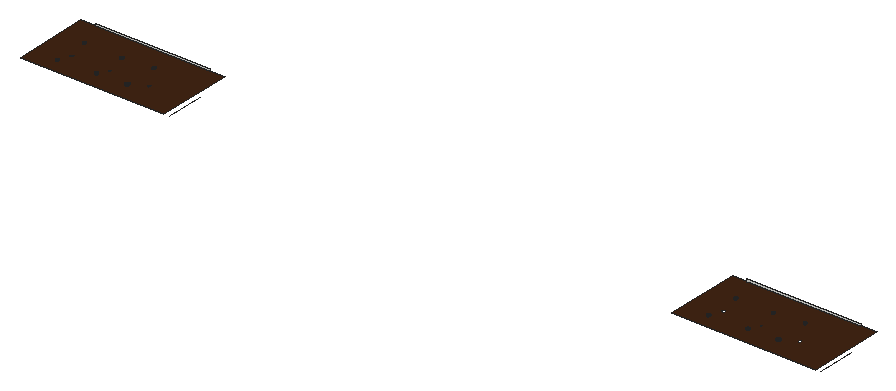
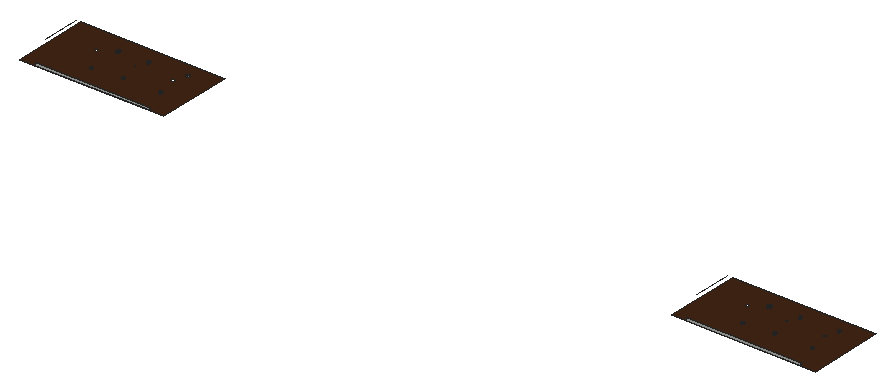
# SketchUp Ruby script. Lengths in inches.
U = 1.inch
M = Sketchup.active_model
def pt(a) = Geom::Point3d.new(a.map { |v| v * U })
def face(e, loops, mat)
  f = e.add_face(loops[0].map { |a| pt(a) })
  loops[1..].each { |l| e.add_face(l.map { |a| pt(a) }).erase! }
  f.material = f.back_material = mat if mat
  f
end
# faces: each face lists its corners as indices into pts; further lists are holes
def faces(e, pts, list, mat = nil) = list.each { |f| face(e, (f[0].is_a?(Array) ? f : [f]).map { |l| l.map { |i| pts[i] } }, mat) }
# xy, xz, yz: faces in a plane at the given z, y or x. An outline is a flat list of corners, or four numbers for a rectangle; further outlines are holes
def ring(l) = l.size == 4 ? [[l[0], l[1]], [l[2], l[1]], [l[2], l[3]], [l[0], l[3]]] : l.each_slice(2).to_a
def flat(e, list, mat, &to3) = list.each { |f| face(e, (f[0].is_a?(Array) ? f : [f]).map { |l| ring(l).map { |u, v| to3.(u, v) } }, mat) }
def xy(e, z, list, mat = nil) = flat(e, list, mat) { |x, y| [x, y, z] }
def xz(e, y, list, mat = nil) = flat(e, list, mat) { |x, z| [x, y, z] }
def yz(e, x, list, mat = nil) = flat(e, list, mat) { |y, z| [x, y, z] }
def lines(e, pts, list) = list.each { |a, b| e.add_line(pt(pts[a]), pt(pts[b])) }
# prism: a flat outline (further loops are holes) pulled along v
def prism(e, loops, v, mat = nil)
  f = face(e, loops, mat); d = Geom::Vector3d.new(v.map { |x| x * U })
  f.pushpull(f.normal.samedirection?(d) ? d.length : -d.length)
end
def box(e, o, s, mat = nil) = prism(e, [[o, [o[0] + s[0], o[1], o[2]], [o[0] + s[0], o[1] + s[1], o[2]], [o[0], o[1] + s[1], o[2]]]], [0, 0, s[2]], mat)
def at(x, y, z, deg = 0) = Geom::Transformation.translation(pt([x, y, z])) * Geom::Transformation.rotation(ORIGIN, Z_AXIS, deg.degrees)
def axes(o, x, y, z) = Geom::Transformation.new([*x, 0, *y, 0, *z, 0, *pt(o).to_a, 1])
def part(name) = M.definitions.add(name)
# library, detail: a bought-in or finely detailed component or shape, given as its bounding box
def library(name, o, s) = part(name).tap { |d| box(d.entities, o, s) }
def detail(e, o, s) = box(e.add_group.entities, o, s)
def put(e, d, t, mat = nil) = e.add_instance(d, t).tap { |i| i.material = mat if mat }
def group(e, t, mat = nil) = e.add_group.tap { |g| g.transformation = t; g.material = mat if mat }.entities
root = M.entities
M.materials.add("[Field Square Tile]").color = [211, 167, 108]
M.materials.add("[Wood Veneer 01]").color = [66, 38, 20]
xy(root,251.5,[[[232.96,2294.125,427.1,2396.68],[273.1,2327.89,273.89,2328,274.63,2328.3,275.26,2328.79,275.75,2329.43,276.06,2330.16,276.16,2330.96,276.06,2331.75,275.75,2332.49,275.26,2333.12,274.63,2333.61,273.89,2333.91,273.1,2334.02,272.31,2333.91,271.57,2333.61,270.93,2333.12,270.45,2332.49,270.14,2331.75,270.04,2330.96,270.14,2330.16,270.45,2329.43,270.93,2328.79,271.57,2328.3,272.31,2328],[377.04,2328.21,377.75,2328.3,378.42,2328.57,378.99,2329.01,379.42,2329.58,379.7,2330.24,379.79,2330.96,379.7,2331.67,379.42,2332.33,378.99,2332.9,378.42,2333.34,377.75,2333.61,377.04,2333.71,376.33,2333.61,375.67,2333.34,375.1,2332.9,374.66,2332.33,374.39,2331.67,374.29,2330.96,374.39,2330.24,374.66,2329.58,375.1,2329.01,375.67,2328.57,376.33,2328.3],[324.47,2328.39,325.13,2328.48,325.75,2328.74,326.28,2329.14,326.69,2329.68,326.95,2330.29,327.03,2330.96,326.95,2331.62,326.69,2332.24,326.28,2332.77,325.75,2333.18,325.13,2333.43,324.47,2333.52,323.81,2333.43,323.19,2333.18,322.66,2332.77,322.25,2332.24,322,2331.62,321.91,2330.96,322,2330.29,322.25,2329.68,322.66,2329.14,323.19,2328.74,323.81,2328.48],[357.2,2316.65,357.83,2316.73,358.42,2316.97,358.92,2317.36,359.31,2317.87,359.55,2318.45,359.63,2319.08,359.55,2319.72,359.31,2320.3,358.92,2320.81,358.42,2321.2,357.83,2321.4375,357.2,2321.52,356.57,2321.4375,355.98,2321.2,355.47,2320.81,355.09,2320.3,354.84,2319.72,354.76,2319.08,354.84,2318.45,355.09,2317.87,355.47,2317.36,355.98,2316.97,356.57,2316.73],[266.8,2358.2,267.28,2358.27,267.74,2358.46,268.125,2358.75,268.42,2359.14,268.61,2359.59,268.67,2360.08,268.61,2360.56,268.42,2361.02,268.125,2361.41,267.74,2361.7,267.28,2361.89,266.8,2361.95,266.3125,2361.89,265.86,2361.7,265.47,2361.41,265.17,2361.02,264.99,2360.56,264.92,2360.08,264.99,2359.59,265.17,2359.14,265.47,2358.75,265.86,2358.46,266.3125,2358.27],[317.24,2358.2,317.72,2358.27,318.17,2358.46,318.5625,2358.75,318.86,2359.14,319.05,2359.59,319.11,2360.08,319.05,2360.56,318.86,2361.02,318.5625,2361.41,318.17,2361.7,317.72,2361.89,317.24,2361.95,316.75,2361.89,316.3,2361.7,315.91,2361.41,315.61,2361.02,315.42,2360.56,315.36,2360.08,315.42,2359.59,315.61,2359.14,315.91,2358.75,316.3,2358.46,316.75,2358.27],[317.24,2315.39,317.72,2315.46,318.17,2315.64,318.5625,2315.94,318.86,2316.33,319.05,2316.78,319.11,2317.27,319.05,2317.75,318.86,2318.2,318.5625,2318.59,318.17,2318.89,317.72,2319.08,317.24,2319.14,316.75,2319.08,316.3,2318.89,315.91,2318.59,315.61,2318.2,315.42,2317.75,315.36,2317.27,315.42,2316.78,315.61,2316.33,315.91,2315.94,316.3,2315.64,316.75,2315.46],[266.8,2312.27,267.28,2312.33,267.74,2312.52,268.125,2312.82,268.42,2313.2,268.61,2313.66,268.67,2314.14,268.61,2314.63,268.42,2315.08,268.125,2315.47,267.74,2315.77,267.28,2315.95,266.8,2316.02,266.3125,2315.95,265.86,2315.77,265.47,2315.47,265.17,2315.08,264.99,2314.63,264.92,2314.14,264.99,2313.66,265.17,2313.2,265.47,2312.82,265.86,2312.52,266.3125,2312.33],[357.2,2362.38,357.63,2362.4375,358.04,2362.6,358.39,2362.87,358.66,2363.22,358.83,2363.63,358.88,2364.07,358.83,2364.5,358.66,2364.91,358.39,2365.26,358.04,2365.53,357.63,2365.7,357.2,2365.75,356.76,2365.7,356.35,2365.53,356,2365.26,355.74,2364.91,355.57,2364.5,355.51,2364.07,355.57,2363.63,355.74,2363.22,356,2362.87,356.35,2362.6,356.76,2362.4375]],[[1111.71,2294.125,1305.85,2396.68],[1151.85,2327.89,1152.64,2328,1153.38,2328.3,1154.01,2328.79,1154.5,2329.43,1154.81,2330.16,1154.91,2330.96,1154.81,2331.75,1154.5,2332.49,1154.01,2333.12,1153.38,2333.61,1152.64,2333.91,1151.85,2334.02,1151.06,2333.91,1150.32,2333.61,1149.68,2333.12,1149.2,2332.49,1148.89,2331.75,1148.79,2330.96,1148.89,2330.16,1149.2,2329.43,1149.68,2328.79,1150.32,2328.3,1151.06,2328],[1255.79,2328.21,1256.5,2328.3,1257.17,2328.57,1257.74,2329.01,1258.17,2329.58,1258.45,2330.24,1258.54,2330.96,1258.45,2331.67,1258.17,2332.33,1257.74,2332.9,1257.17,2333.34,1256.5,2333.61,1255.79,2333.71,1255.08,2333.61,1254.42,2333.34,1253.85,2332.9,1253.41,2332.33,1253.14,2331.67,1253.04,2330.96,1253.14,2330.24,1253.41,2329.58,1253.85,2329.01,1254.42,2328.57,1255.08,2328.3],[1203.22,2328.39,1203.88,2328.48,1204.5,2328.74,1205.03,2329.14,1205.44,2329.68,1205.7,2330.29,1205.78,2330.96,1205.7,2331.62,1205.44,2332.24,1205.03,2332.77,1204.5,2333.18,1203.88,2333.43,1203.22,2333.52,1202.56,2333.43,1201.94,2333.18,1201.41,2332.77,1201,2332.24,1200.75,2331.62,1200.66,2330.96,1200.75,2330.29,1201,2329.68,1201.41,2329.14,1201.94,2328.74,1202.56,2328.48],[1235.95,2316.65,1236.58,2316.73,1237.17,2316.97,1237.67,2317.36,1238.06,2317.87,1238.3,2318.45,1238.38,2319.08,1238.3,2319.72,1238.06,2320.3,1237.67,2320.81,1237.17,2321.2,1236.58,2321.4375,1235.95,2321.52,1235.32,2321.4375,1234.73,2321.2,1234.22,2320.81,1233.84,2320.3,1233.59,2319.72,1233.51,2319.08,1233.59,2318.45,1233.84,2317.87,1234.22,2317.36,1234.73,2316.97,1235.32,2316.73],[1145.55,2358.2,1146.03,2358.27,1146.49,2358.46,1146.875,2358.75,1147.17,2359.14,1147.36,2359.59,1147.42,2360.08,1147.36,2360.56,1147.17,2361.02,1146.875,2361.41,1146.49,2361.7,1146.03,2361.89,1145.55,2361.95,1145.0625,2361.89,1144.61,2361.7,1144.22,2361.41,1143.92,2361.02,1143.74,2360.56,1143.67,2360.08,1143.74,2359.59,1143.92,2359.14,1144.22,2358.75,1144.61,2358.46,1145.0625,2358.27],[1195.99,2358.2,1196.47,2358.27,1196.92,2358.46,1197.3125,2358.75,1197.61,2359.14,1197.8,2359.59,1197.86,2360.08,1197.8,2360.56,1197.61,2361.02,1197.3125,2361.41,1196.92,2361.7,1196.47,2361.89,1195.99,2361.95,1195.5,2361.89,1195.05,2361.7,1194.66,2361.41,1194.36,2361.02,1194.17,2360.56,1194.11,2360.08,1194.17,2359.59,1194.36,2359.14,1194.66,2358.75,1195.05,2358.46,1195.5,2358.27],[1195.99,2315.39,1196.47,2315.46,1196.92,2315.64,1197.3125,2315.94,1197.61,2316.33,1197.8,2316.78,1197.86,2317.27,1197.8,2317.75,1197.61,2318.2,1197.3125,2318.59,1196.92,2318.89,1196.47,2319.08,1195.99,2319.14,1195.5,2319.08,1195.05,2318.89,1194.66,2318.59,1194.36,2318.2,1194.17,2317.75,1194.11,2317.27,1194.17,2316.78,1194.36,2316.33,1194.66,2315.94,1195.05,2315.64,1195.5,2315.46],[1145.55,2312.27,1146.03,2312.33,1146.49,2312.52,1146.875,2312.82,1147.17,2313.2,1147.36,2313.66,1147.42,2314.14,1147.36,2314.63,1147.17,2315.08,1146.875,2315.47,1146.49,2315.77,1146.03,2315.95,1145.55,2316.02,1145.0625,2315.95,1144.61,2315.77,1144.22,2315.47,1143.92,2315.08,1143.74,2314.63,1143.67,2314.14,1143.74,2313.66,1143.92,2313.2,1144.22,2312.82,1144.61,2312.52,1145.0625,2312.33],[1235.95,2362.38,1236.38,2362.4375,1236.79,2362.6,1237.14,2362.87,1237.41,2363.22,1237.58,2363.63,1237.63,2364.07,1237.58,2364.5,1237.41,2364.91,1237.14,2365.26,1236.79,2365.53,1236.38,2365.7,1235.95,2365.75,1235.51,2365.7,1235.1,2365.53,1234.75,2365.26,1234.49,2364.91,1234.32,2364.5,1234.26,2364.07,1234.32,2363.63,1234.49,2363.22,1234.75,2362.87,1235.1,2362.6,1235.51,2362.4375]]],"[Wood Veneer 01]")
xz(root,2396.68,[[252.78,251.5,252.84,254.5],[252.84,251.5,406.85,254.5],[1131.53,251.5,1131.59,254.5],[1131.59,251.5,1285.6,254.5]])
p = [[266.3125,2312.33,251.5],[265.86,2312.52,251.5],[265.86,2312.52,252.5],[266.3125,2312.33,252.5],[266.8,2312.27,251.5],[266.8,2312.27,252.5],
  [267.28,2312.33,251.5],[267.28,2312.33,252.5],[267.74,2312.52,251.5],[267.74,2312.52,252.5],[1145.0625,2312.33,251.5],[1144.61,2312.52,251.5],
  [1144.61,2312.52,252.5],[1145.0625,2312.33,252.5],[1145.55,2312.27,251.5],[1145.55,2312.27,252.5],[1146.03,2312.33,251.5],[1146.03,2312.33,252.5],
  [1146.49,2312.52,251.5],[1146.49,2312.52,252.5],[265.47,2312.82,251.5],[265.47,2312.82,252.5],[268.125,2312.82,251.5],[268.125,2312.82,252.5],
  [1144.22,2312.82,251.5],[1144.22,2312.82,252.5],[1146.875,2312.82,251.5],[1146.875,2312.82,252.5],[265.17,2313.2,251.5],[265.17,2313.2,252.5],
  [268.42,2313.2,251.5],[268.42,2313.2,252.5],[1143.92,2313.2,251.5],[1143.92,2313.2,252.5],[1147.17,2313.2,251.5],[1147.17,2313.2,252.5],
  [264.99,2313.66,251.5],[264.99,2313.66,252.5],[268.61,2313.66,251.5],[268.61,2313.66,252.5],[1143.74,2313.66,251.5],[1143.74,2313.66,252.5],
  [1147.36,2313.66,251.5],[1147.36,2313.66,252.5],[264.92,2314.14,251.5],[264.92,2314.14,252.5],[268.67,2314.14,251.5],[268.67,2314.14,252.5],
  [1143.67,2314.14,251.5],[1143.67,2314.14,252.5],[1147.42,2314.14,251.5],[1147.42,2314.14,252.5],[264.99,2314.63,251.5],[264.99,2314.63,252.5],
  [268.61,2314.63,251.5],[268.61,2314.63,252.5],[1143.74,2314.63,251.5],[1143.74,2314.63,252.5],[1147.36,2314.63,251.5],[1147.36,2314.63,252.5],
  [265.17,2315.08,251.5],[265.17,2315.08,252.5],[268.42,2315.08,251.5],[268.42,2315.08,252.5],[1143.92,2315.08,251.5],[1143.92,2315.08,252.5],
  [1147.17,2315.08,251.5],[1147.17,2315.08,252.5],[265.47,2315.47,251.5],[265.47,2315.47,252.5],[268.125,2315.47,251.5],[268.125,2315.47,252.5],
  [1144.22,2315.47,251.5],[1144.22,2315.47,252.5],[1146.875,2315.47,251.5],[1146.875,2315.47,252.5],[317.24,2315.39,251.5],[316.75,2315.46,251.5],
  [316.75,2315.46,252.5],[317.24,2315.39,252.5],[317.72,2315.46,251.5],[317.72,2315.46,252.5],[1195.99,2315.39,251.5],[1195.5,2315.46,251.5],
  [1195.5,2315.46,252.5],[1195.99,2315.39,252.5],[1196.47,2315.46,251.5],[1196.47,2315.46,252.5],[265.86,2315.77,251.5],[265.86,2315.77,252.5],
  [267.74,2315.77,251.5],[267.74,2315.77,252.5],[316.3,2315.64,251.5],[316.3,2315.64,252.5],[318.17,2315.64,251.5],[318.17,2315.64,252.5],
  [1144.61,2315.77,251.5],[1144.61,2315.77,252.5],[1146.49,2315.77,251.5],[1146.49,2315.77,252.5],[1195.05,2315.64,251.5],[1195.05,2315.64,252.5],
  [1196.92,2315.64,251.5],[1196.92,2315.64,252.5],[315.91,2315.94,251.5],[315.91,2315.94,252.5],[318.5625,2315.94,251.5],[318.5625,2315.94,252.5],
  [1194.66,2315.94,251.5],[1194.66,2315.94,252.5],[1197.3125,2315.94,251.5],[1197.3125,2315.94,252.5],[266.3125,2315.95,251.5],[266.3125,2315.95,252.5],
  [267.28,2315.95,251.5],[267.28,2315.95,252.5],[1145.0625,2315.95,251.5],[1145.0625,2315.95,252.5],[1146.03,2315.95,251.5],[1146.03,2315.95,252.5],
  [315.61,2316.33,251.5],[315.61,2316.33,252.5],[318.86,2316.33,251.5],[318.86,2316.33,252.5],[1194.36,2316.33,251.5],[1194.36,2316.33,252.5],
  [1197.61,2316.33,251.5],[1197.61,2316.33,252.5],[266.8,2316.02,251.5],[266.8,2316.02,252.5],[1145.55,2316.02,251.5],[1145.55,2316.02,252.5],
  [315.42,2316.78,251.5],[315.42,2316.78,252.5],[319.05,2316.78,251.5],[319.05,2316.78,252.5],[1194.17,2316.78,251.5],[1194.17,2316.78,252.5],
  [1197.8,2316.78,251.5],[1197.8,2316.78,252.5],[357.2,2316.65,251.5],[356.57,2316.73,251.5],[356.57,2316.73,252.5625],[357.2,2316.65,252.5625],
  [357.83,2316.73,251.5],[357.83,2316.73,252.5625],[1235.95,2316.65,251.5],[1235.32,2316.73,251.5],[1235.32,2316.73,252.5625],[1235.95,2316.65,252.5625],
  [1236.58,2316.73,251.5],[1236.58,2316.73,252.5625],[355.98,2316.97,251.5],[355.98,2316.97,252.5625],[358.42,2316.97,251.5],[358.42,2316.97,252.5625],
  [1234.73,2316.97,251.5],[1234.73,2316.97,252.5625],[1237.17,2316.97,251.5],[1237.17,2316.97,252.5625],[315.36,2317.27,251.5],[315.36,2317.27,252.5],
  [319.11,2317.27,251.5],[319.11,2317.27,252.5],[1194.11,2317.27,251.5],[1194.11,2317.27,252.5],[1197.86,2317.27,251.5],[1197.86,2317.27,252.5],
  [355.47,2317.36,251.5],[355.47,2317.36,252.5625],[358.92,2317.36,251.5],[358.92,2317.36,252.5625],[1234.22,2317.36,251.5],[1234.22,2317.36,252.5625],
  [1237.67,2317.36,251.5],[1237.67,2317.36,252.5625],[315.42,2317.75,251.5],[315.42,2317.75,252.5],[319.05,2317.75,251.5],[319.05,2317.75,252.5],
  [1194.17,2317.75,251.5],[1194.17,2317.75,252.5],[1197.8,2317.75,251.5],[1197.8,2317.75,252.5],[355.09,2317.87,251.5],[355.09,2317.87,252.5625],
  [359.31,2317.87,251.5],[359.31,2317.87,252.5625],[1233.84,2317.87,251.5],[1233.84,2317.87,252.5625],[1238.06,2317.87,251.5],[1238.06,2317.87,252.5625],
  [315.61,2318.2,251.5],[315.61,2318.2,252.5],[318.86,2318.2,251.5],[318.86,2318.2,252.5],[1194.36,2318.2,251.5],[1194.36,2318.2,252.5],
  [1197.61,2318.2,251.5],[1197.61,2318.2,252.5],[354.84,2318.45,251.5],[354.84,2318.45,252.5625],[359.55,2318.45,251.5],[359.55,2318.45,252.5625],
  [1233.59,2318.45,251.5],[1233.59,2318.45,252.5625],[1238.3,2318.45,251.5],[1238.3,2318.45,252.5625],[315.91,2318.59,251.5],[315.91,2318.59,252.5],
  [318.5625,2318.59,251.5],[318.5625,2318.59,252.5],[1194.66,2318.59,251.5],[1194.66,2318.59,252.5],[1197.3125,2318.59,251.5],[1197.3125,2318.59,252.5],
  [354.76,2319.08,251.5],[354.76,2319.08,252.5625],[359.63,2319.08,251.5],[359.63,2319.08,252.5625],[1233.51,2319.08,251.5],[1233.51,2319.08,252.5625],
  [1238.38,2319.08,251.5],[1238.38,2319.08,252.5625],[316.3,2318.89,251.5],[316.3,2318.89,252.5],[318.17,2318.89,251.5],[318.17,2318.89,252.5],
  [1195.05,2318.89,251.5],[1195.05,2318.89,252.5],[1196.92,2318.89,251.5],[1196.92,2318.89,252.5],[316.75,2319.08,251.5],[316.75,2319.08,252.5],
  [317.72,2319.08,251.5],[317.72,2319.08,252.5],[1195.5,2319.08,251.5],[1195.5,2319.08,252.5],[1196.47,2319.08,251.5],[1196.47,2319.08,252.5],
  [317.24,2319.14,251.5],[317.24,2319.14,252.5],[354.84,2319.72,251.5],[354.84,2319.72,252.5625],[359.55,2319.72,251.5],[359.55,2319.72,252.5625],
  [1195.99,2319.14,251.5],[1195.99,2319.14,252.5],[1233.59,2319.72,251.5],[1233.59,2319.72,252.5625],[1238.3,2319.72,251.5],[1238.3,2319.72,252.5625],
  [355.09,2320.3,251.5],[355.09,2320.3,252.5625],[359.31,2320.3,251.5],[359.31,2320.3,252.5625],[1233.84,2320.3,251.5],[1233.84,2320.3,252.5625],
  [1238.06,2320.3,251.5],[1238.06,2320.3,252.5625],[355.47,2320.81,251.5],[355.47,2320.81,252.5625],[358.92,2320.81,251.5],[358.92,2320.81,252.5625],
  [1234.22,2320.81,251.5],[1234.22,2320.81,252.5625],[1237.67,2320.81,251.5],[1237.67,2320.81,252.5625],[355.98,2321.2,251.5],[355.98,2321.2,252.5625],
  [358.42,2321.2,251.5],[358.42,2321.2,252.5625],[1234.73,2321.2,251.5],[1234.73,2321.2,252.5625],[1237.17,2321.2,251.5],[1237.17,2321.2,252.5625],
  [356.57,2321.4375,251.5],[356.57,2321.4375,252.5625],[357.83,2321.4375,251.5],[357.83,2321.4375,252.5625],[1235.32,2321.4375,251.5],[1235.32,2321.4375,252.5625],
  [1236.58,2321.4375,251.5],[1236.58,2321.4375,252.5625],[357.2,2321.52,251.5],[357.2,2321.52,252.5625],[1235.95,2321.52,251.5],[1235.95,2321.52,252.5625],
  [266.8,2358.2,251.5],[266.3125,2358.27,251.5],[266.3125,2358.27,252.5],[266.8,2358.2,252.5],[267.28,2358.27,251.5],[267.28,2358.27,252.5],
  [317.24,2358.2,251.5],[316.75,2358.27,251.5],[316.75,2358.27,252.5],[317.24,2358.2,252.5],[317.72,2358.27,251.5],[317.72,2358.27,252.5],
  [1145.55,2358.2,251.5],[1145.0625,2358.27,251.5],[1145.0625,2358.27,252.5],[1145.55,2358.2,252.5],[1146.03,2358.27,251.5],[1146.03,2358.27,252.5],
  [1195.99,2358.2,251.5],[1195.5,2358.27,251.5],[1195.5,2358.27,252.5],[1195.99,2358.2,252.5],[1196.47,2358.27,251.5],[1196.47,2358.27,252.5],
  [265.86,2358.46,251.5],[265.86,2358.46,252.5],[267.74,2358.46,251.5],[267.74,2358.46,252.5],[316.3,2358.46,251.5],[316.3,2358.46,252.5],
  [318.17,2358.46,251.5],[318.17,2358.46,252.5],[1144.61,2358.46,251.5],[1144.61,2358.46,252.5],[1146.49,2358.46,251.5],[1146.49,2358.46,252.5],
  [1195.05,2358.46,251.5],[1195.05,2358.46,252.5],[1196.92,2358.46,251.5],[1196.92,2358.46,252.5],[265.47,2358.75,251.5],[265.47,2358.75,252.5],
  [268.125,2358.75,251.5],[268.125,2358.75,252.5],[315.91,2358.75,251.5],[315.91,2358.75,252.5],[318.5625,2358.75,251.5],[318.5625,2358.75,252.5],
  [1144.22,2358.75,251.5],[1144.22,2358.75,252.5],[1146.875,2358.75,251.5],[1146.875,2358.75,252.5],[1194.66,2358.75,251.5],[1194.66,2358.75,252.5],
  [1197.3125,2358.75,251.5],[1197.3125,2358.75,252.5],[265.17,2359.14,251.5],[265.17,2359.14,252.5],[268.42,2359.14,251.5],[268.42,2359.14,252.5],
  [315.61,2359.14,251.5],[315.61,2359.14,252.5],[318.86,2359.14,251.5],[318.86,2359.14,252.5],[1143.92,2359.14,251.5],[1143.92,2359.14,252.5],
  [1147.17,2359.14,251.5],[1147.17,2359.14,252.5],[1194.36,2359.14,251.5],[1194.36,2359.14,252.5],[1197.61,2359.14,251.5],[1197.61,2359.14,252.5],
  [264.99,2359.59,251.5],[264.99,2359.59,252.5],[268.61,2359.59,251.5],[268.61,2359.59,252.5],[315.42,2359.59,251.5],[315.42,2359.59,252.5],
  [319.05,2359.59,251.5],[319.05,2359.59,252.5],[1143.74,2359.59,251.5],[1143.74,2359.59,252.5],[1147.36,2359.59,251.5],[1147.36,2359.59,252.5],
  [1194.17,2359.59,251.5],[1194.17,2359.59,252.5],[1197.8,2359.59,251.5],[1197.8,2359.59,252.5],[264.92,2360.08,251.5],[264.92,2360.08,252.5],
  [268.67,2360.08,251.5],[268.67,2360.08,252.5],[315.36,2360.08,251.5],[315.36,2360.08,252.5],[319.11,2360.08,251.5],[319.11,2360.08,252.5],
  [1143.67,2360.08,251.5],[1143.67,2360.08,252.5],[1147.42,2360.08,251.5],[1147.42,2360.08,252.5],[1194.11,2360.08,251.5],[1194.11,2360.08,252.5],
  [1197.86,2360.08,251.5],[1197.86,2360.08,252.5],[264.99,2360.56,251.5],[264.99,2360.56,252.5],[268.61,2360.56,251.5],[268.61,2360.56,252.5],
  [315.42,2360.56,251.5],[315.42,2360.56,252.5],[319.05,2360.56,251.5],[319.05,2360.56,252.5],[1143.74,2360.56,251.5],[1143.74,2360.56,252.5],
  [1147.36,2360.56,251.5],[1147.36,2360.56,252.5],[1194.17,2360.56,251.5],[1194.17,2360.56,252.5],[1197.8,2360.56,251.5],[1197.8,2360.56,252.5],
  [265.17,2361.02,251.5],[265.17,2361.02,252.5],[268.42,2361.02,251.5],[268.42,2361.02,252.5],[315.61,2361.02,251.5],[315.61,2361.02,252.5],
  [318.86,2361.02,251.5],[318.86,2361.02,252.5],[1143.92,2361.02,251.5],[1143.92,2361.02,252.5],[1147.17,2361.02,251.5],[1147.17,2361.02,252.5],
  [1194.36,2361.02,251.5],[1194.36,2361.02,252.5],[1197.61,2361.02,251.5],[1197.61,2361.02,252.5],[265.47,2361.41,251.5],[265.47,2361.41,252.5],
  [268.125,2361.41,251.5],[268.125,2361.41,252.5],[315.91,2361.41,251.5],[315.91,2361.41,252.5],[318.5625,2361.41,251.5],[318.5625,2361.41,252.5],
  [1144.22,2361.41,251.5],[1144.22,2361.41,252.5],[1146.875,2361.41,251.5],[1146.875,2361.41,252.5],[1194.66,2361.41,251.5],[1194.66,2361.41,252.5],
  [1197.3125,2361.41,251.5],[1197.3125,2361.41,252.5],[265.86,2361.7,251.5],[265.86,2361.7,252.5],[267.74,2361.7,251.5],[267.74,2361.7,252.5],
  [316.3,2361.7,251.5],[316.3,2361.7,252.5],[318.17,2361.7,251.5],[318.17,2361.7,252.5],[1144.61,2361.7,251.5],[1144.61,2361.7,252.5],
  [1146.49,2361.7,251.5],[1146.49,2361.7,252.5],[1195.05,2361.7,251.5],[1195.05,2361.7,252.5],[1196.92,2361.7,251.5],[1196.92,2361.7,252.5],
  [266.3125,2361.89,251.5],[266.3125,2361.89,252.5],[267.28,2361.89,251.5],[267.28,2361.89,252.5],[316.75,2361.89,251.5],[316.75,2361.89,252.5],
  [317.72,2361.89,251.5],[317.72,2361.89,252.5],[1145.0625,2361.89,251.5],[1145.0625,2361.89,252.5],[1146.03,2361.89,251.5],[1146.03,2361.89,252.5],
  [1195.5,2361.89,251.5],[1195.5,2361.89,252.5],[1196.47,2361.89,251.5],[1196.47,2361.89,252.5],[266.8,2361.95,251.5],[266.8,2361.95,252.5],
  [317.24,2361.95,251.5],[317.24,2361.95,252.5],[1145.55,2361.95,251.5],[1145.55,2361.95,252.5],[1195.99,2361.95,251.5],[1195.99,2361.95,252.5],
  [356.76,2362.4375,251.5],[356.35,2362.6,251.5],[356.35,2362.6,252.4375],[356.76,2362.4375,252.4375],[357.2,2362.38,251.5],[357.2,2362.38,252.4375],
  [357.63,2362.4375,251.5],[357.63,2362.4375,252.4375],[358.04,2362.6,251.5],[358.04,2362.6,252.4375],[1235.51,2362.4375,251.5],[1235.1,2362.6,251.5],
  [1235.1,2362.6,252.4375],[1235.51,2362.4375,252.4375],[1235.95,2362.38,251.5],[1235.95,2362.38,252.4375],[1236.38,2362.4375,251.5],[1236.38,2362.4375,252.4375],
  [1236.79,2362.6,251.5],[1236.79,2362.6,252.4375],[356,2362.87,251.5],[356,2362.87,252.4375],[358.39,2362.87,251.5],[358.39,2362.87,252.4375],
  [1234.75,2362.87,251.5],[1234.75,2362.87,252.4375],[1237.14,2362.87,251.5],[1237.14,2362.87,252.4375],[355.74,2363.22,251.5],[355.74,2363.22,252.4375],
  [358.66,2363.22,251.5],[358.66,2363.22,252.4375],[1234.49,2363.22,251.5],[1234.49,2363.22,252.4375],[1237.41,2363.22,251.5],[1237.41,2363.22,252.4375],
  [355.57,2363.63,251.5],[355.57,2363.63,252.4375],[358.83,2363.63,251.5],[358.83,2363.63,252.4375],[1234.32,2363.63,251.5],[1234.32,2363.63,252.4375],
  [1237.58,2363.63,251.5],[1237.58,2363.63,252.4375],[355.51,2364.07,251.5],[355.51,2364.07,252.4375],[358.88,2364.07,251.5],[358.88,2364.07,252.4375],
  [1234.26,2364.07,251.5],[1234.26,2364.07,252.4375],[1237.63,2364.07,251.5],[1237.63,2364.07,252.4375],[355.57,2364.5,251.5],[355.57,2364.5,252.4375],
  [358.83,2364.5,251.5],[358.83,2364.5,252.4375],[1234.32,2364.5,251.5],[1234.32,2364.5,252.4375],[1237.58,2364.5,251.5],[1237.58,2364.5,252.4375],
  [355.74,2364.91,251.5],[355.74,2364.91,252.4375],[358.66,2364.91,251.5],[358.66,2364.91,252.4375],[1234.49,2364.91,251.5],[1234.49,2364.91,252.4375],
  [1237.41,2364.91,251.5],[1237.41,2364.91,252.4375],[356,2365.26,251.5],[356,2365.26,252.4375],[358.39,2365.26,251.5],[358.39,2365.26,252.4375],
  [1234.75,2365.26,251.5],[1234.75,2365.26,252.4375],[1237.14,2365.26,251.5],[1237.14,2365.26,252.4375],[356.35,2365.53,251.5],[356.35,2365.53,252.4375],
  [358.04,2365.53,251.5],[358.04,2365.53,252.4375],[1235.1,2365.53,251.5],[1235.1,2365.53,252.4375],[1236.79,2365.53,251.5],[1236.79,2365.53,252.4375],
  [356.76,2365.7,251.5],[356.76,2365.7,252.4375],[357.63,2365.7,251.5],[357.63,2365.7,252.4375],[1235.51,2365.7,251.5],[1235.51,2365.7,252.4375],
  [1236.38,2365.7,251.5],[1236.38,2365.7,252.4375],[357.2,2365.75,251.5],[357.2,2365.75,252.4375],[1235.95,2365.75,251.5],[1235.95,2365.75,252.4375],
  [433.97,2346.71,251.5],[433.97,2294.125,251.5],[1312.72,2346.71,251.5],[1312.72,2294.125,251.5]]
faces(root,p,[[0,1,2,3],[4,0,3,5],[6,4,5,7],[8,6,7,9],[10,11,12,13],[14,10,13,15],[16,14,15,17],[18,16,17,19],
  [1,20,21,2],[22,8,9,23],[11,24,25,12],[26,18,19,27],[20,28,29,21],[30,22,23,31],[24,32,33,25],[34,26,27,35],
  [28,36,37,29],[38,30,31,39],[32,40,41,33],[42,34,35,43],[36,44,45,37],[46,38,39,47],[40,48,49,41],[50,42,43,51],
  [44,52,53,45],[54,46,47,55],[48,56,57,49],[58,50,51,59],[52,60,61,53],[62,54,55,63],[56,64,65,57],[66,58,59,67],
  [60,68,69,61],[70,62,63,71],[64,72,73,65],[74,66,67,75],[76,77,78,79],[80,76,79,81],[82,83,84,85],[86,82,85,87],
  [68,88,89,69],[90,70,71,91],[77,92,93,78],[94,80,81,95],[72,96,97,73],[98,74,75,99],[83,100,101,84],[102,86,87,103],
  [92,104,105,93],[106,94,95,107],[100,108,109,101],[110,102,103,111],[88,112,113,89],[114,90,91,115],[96,116,117,97],[118,98,99,119],
  [104,120,121,105],[122,106,107,123],[108,124,125,109],[126,110,111,127],[112,128,129,113],[128,114,115,129],[116,130,131,117],[130,118,119,131],
  [120,132,133,121],[134,122,123,135],[124,136,137,125],[138,126,127,139],[140,141,142,143],[144,140,143,145],[146,147,148,149],[150,146,149,151],
  [141,152,153,142],[154,144,145,155],[147,156,157,148],[158,150,151,159],[132,160,161,133],[162,134,135,163],[136,164,165,137],[166,138,139,167],
  [152,168,169,153],[170,154,155,171],[156,172,173,157],[174,158,159,175],[160,176,177,161],[178,162,163,179],[164,180,181,165],[182,166,167,183],
  [168,184,185,169],[186,170,171,187],[172,188,189,173],[190,174,175,191],[176,192,193,177],[194,178,179,195],[180,196,197,181],[198,182,183,199],
  [184,200,201,185],[202,186,187,203],[188,204,205,189],[206,190,191,207],[192,208,209,193],[210,194,195,211],[196,212,213,197],[214,198,199,215],
  [200,216,217,201],[218,202,203,219],[204,220,221,205],[222,206,207,223],[208,224,225,209],[226,210,211,227],[212,228,229,213],[230,214,215,231],
  [224,232,233,225],[234,226,227,235],[228,236,237,229],[238,230,231,239],[232,240,241,233],[240,234,235,241],[216,242,243,217],[244,218,219,245],
  [236,246,247,237],[246,238,239,247],[220,248,249,221],[250,222,223,251],[242,252,253,243],[254,244,245,255],[248,256,257,249],[258,250,251,259],
  [252,260,261,253],[262,254,255,263],[256,264,265,257],[266,258,259,267],[260,268,269,261],[270,262,263,271],[264,272,273,265],[274,266,267,275],
  [268,276,277,269],[278,270,271,279],[272,280,281,273],[282,274,275,283],[276,284,285,277],[284,278,279,285],[280,286,287,281],[286,282,283,287],
  [288,289,290,291],[292,288,291,293],[294,295,296,297],[298,294,297,299],[300,301,302,303],[304,300,303,305],[306,307,308,309],[310,306,309,311],
  [289,312,313,290],[314,292,293,315],[295,316,317,296],[318,298,299,319],[301,320,321,302],[322,304,305,323],[307,324,325,308],[326,310,311,327],
  [312,328,329,313],[330,314,315,331],[316,332,333,317],[334,318,319,335],[320,336,337,321],[338,322,323,339],[324,340,341,325],[342,326,327,343],
  [328,344,345,329],[346,330,331,347],[332,348,349,333],[350,334,335,351],[336,352,353,337],[354,338,339,355],[340,356,357,341],[358,342,343,359],
  [344,360,361,345],[362,346,347,363],[348,364,365,349],[366,350,351,367],[352,368,369,353],[370,354,355,371],[356,372,373,357],[374,358,359,375],
  [360,376,377,361],[378,362,363,379],[364,380,381,365],[382,366,367,383],[368,384,385,369],[386,370,371,387],[372,388,389,373],[390,374,375,391],
  [376,392,393,377],[394,378,379,395],[380,396,397,381],[398,382,383,399],[384,400,401,385],[402,386,387,403],[388,404,405,389],[406,390,391,407],
  [392,408,409,393],[410,394,395,411],[396,412,413,397],[414,398,399,415],[400,416,417,401],[418,402,403,419],[404,420,421,405],[422,406,407,423],
  [408,424,425,409],[426,410,411,427],[412,428,429,413],[430,414,415,431],[416,432,433,417],[434,418,419,435],[420,436,437,421],[438,422,423,439],
  [424,440,441,425],[442,426,427,443],[428,444,445,429],[446,430,431,447],[432,448,449,433],[450,434,435,451],[436,452,453,437],[454,438,439,455],
  [440,456,457,441],[458,442,443,459],[444,460,461,445],[462,446,447,463],[448,464,465,449],[466,450,451,467],[452,468,469,453],[470,454,455,471],
  [456,472,473,457],[472,458,459,473],[460,474,475,461],[474,462,463,475],[464,476,477,465],[476,466,467,477],[468,478,479,469],[478,470,471,479],
  [480,481,482,483],[484,480,483,485],[486,484,485,487],[488,486,487,489],[490,491,492,493],[494,490,493,495],[496,494,495,497],[498,496,497,499],
  [481,500,501,482],[502,488,489,503],[491,504,505,492],[506,498,499,507],[500,508,509,501],[510,502,503,511],[504,512,513,505],[514,506,507,515],
  [508,516,517,509],[518,510,511,519],[512,520,521,513],[522,514,515,523],[516,524,525,517],[526,518,519,527],[520,528,529,521],[530,522,523,531],
  [524,532,533,525],[534,526,527,535],[528,536,537,529],[538,530,531,539],[532,540,541,533],[542,534,535,543],[536,544,545,537],[546,538,539,547],
  [540,548,549,541],[550,542,543,551],[544,552,553,545],[554,546,547,555],[548,556,557,549],[558,550,551,559],[552,560,561,553],[562,554,555,563],
  [556,564,565,557],[566,558,559,567],[560,568,569,561],[570,562,563,571],[564,572,573,565],[572,566,567,573],[568,574,575,569],[574,570,571,575]],"[Field Square Tile]")
lines(root,p,[[576,577],[578,579]])
